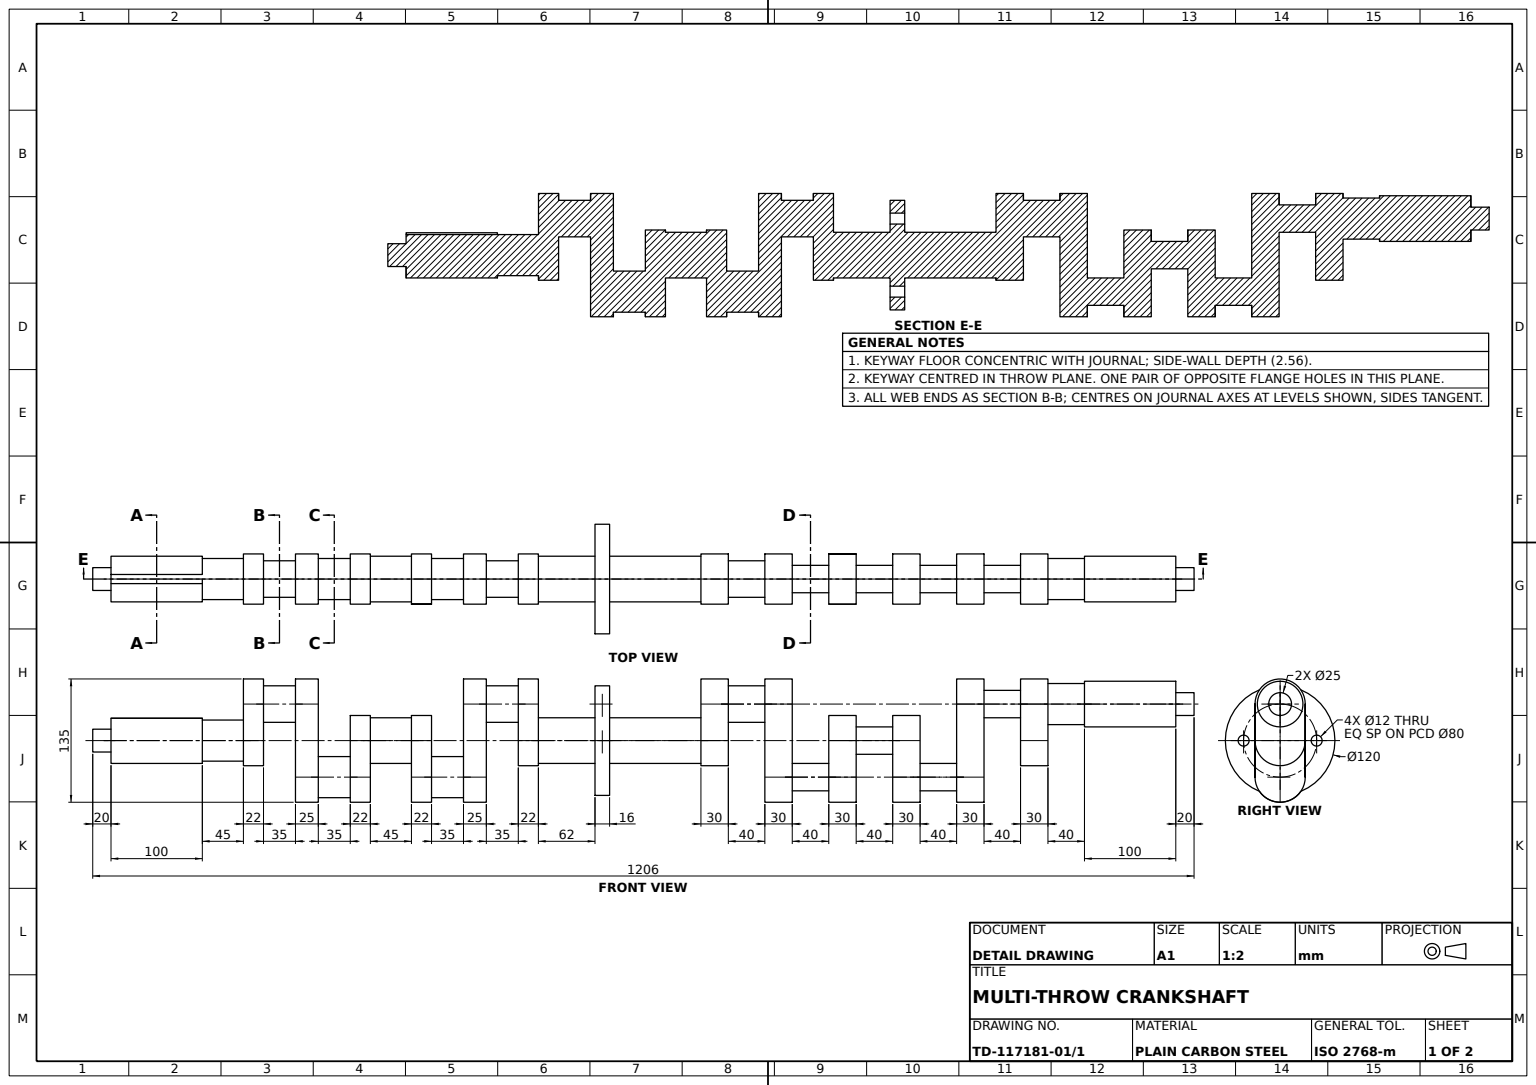
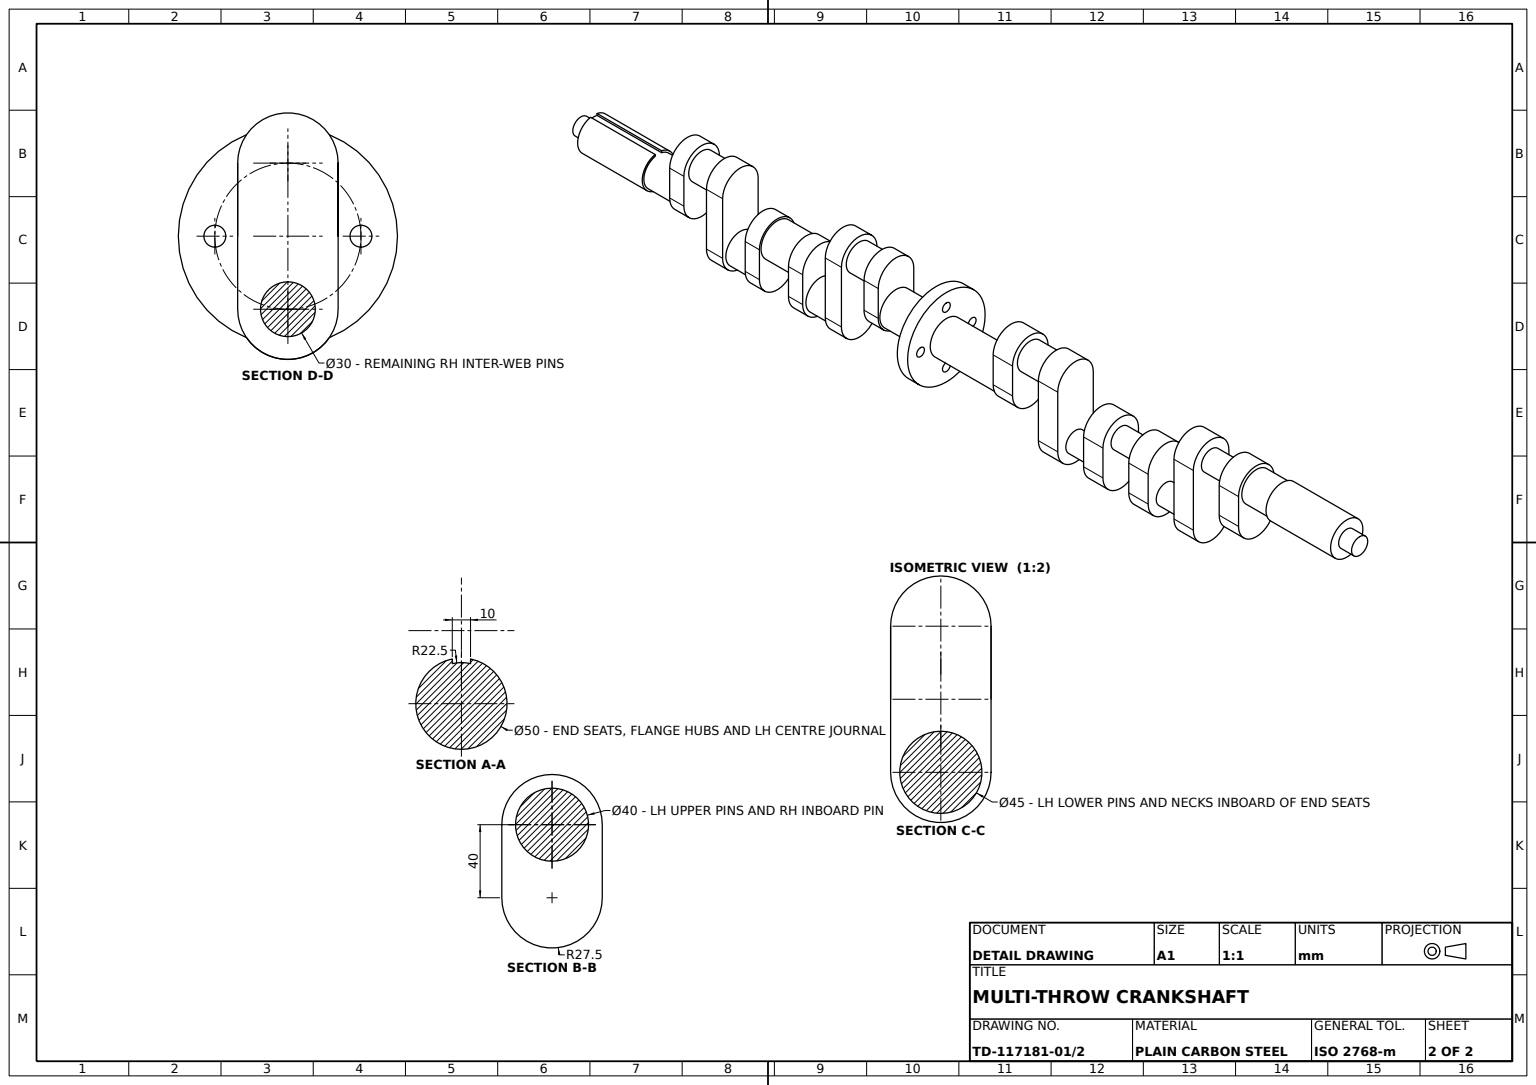
solid
v1 (0,-27.5,-240)
v2 (0,27.5,-240)
e1 v1 v2 CIRCLE(AX(P(0,0,-240),D(0,0,-1),D(-1,0,0)),27.5)
v3 (0,27.5,-270)
e2 v3 v2 LINE
v4 (0,-27.5,-270)
e3 v4 v3 CIRCLE(AX(P(0,0,-270),D(0,0,-1),D(-1,0,0)),27.5)
e4 v4 v1 LINE
face CYL(AX(P(0,0,-270),D(0,0,1),D(1,0,0)),27.5) [e1 -e2 -e3 e4]
v5 (62.5,0,195)
v6 (62.5,0,160)
e5 v5 v6 LINE
v7 (17.5,0,160)
e6 v6 v7 CIRCLE(AX(P(40,0,160),D(0,0,1),D(1,0,0)),22.5)
v8 (17.5,0,195)
e7 v8 v7 LINE
e8 v5 v8 CIRCLE(AX(P(40,0,195),D(0,0,1),D(1,0,0)),22.5)
face CYL(AX(P(40,0,195),D(0,0,-1),D(-1,0,0)),22.5) [e5 e6 -e7 -e8]
v9 (-25,0,-410)
v10 (-55,0,-410)
e9 v9 v10 CIRCLE(AX(P(-40,0,-410),D(0,0,-1),D(-1,0,0)),15)
v11 (-55,0,-450)
e10 v11 v10 LINE
v12 (-25,0,-450)
e11 v12 v11 CIRCLE(AX(P(-40,0,-450),D(0,0,-1),D(-1,0,0)),15)
e12 v12 v9 LINE
face CYL(AX(P(-40,0,-450),D(0,0,1),D(1,0,0)),15) [e9 -e10 -e11 e12]
v13 (-40,27.5,78)
v14 (-67.5,0,78)
e13 v13 v14 CIRCLE(AX(P(-40,0,78),D(0,0,1),D(1,0,0)),27.5)
v15 (-67.5,0,100)
e14 v15 v14 LINE
v16 (-40,27.5,100)
e15 v16 v15 CIRCLE(AX(P(-40,0,100),D(0,0,1),D(1,0,0)),27.5)
e16 v16 v13 LINE
face CYL(AX(P(-40,0,100),D(0,0,-1),D(-1,0,0)),27.5) [e13 -e14 -e15 e16]
v17 (25,0,-240)
v18 (55,0,-240)
e17 v17 v18 CIRCLE(AX(P(40,0,-240),D(0,0,-1),D(-1,0,0)),15)
v19 (25,0,-200)
e18 v17 v19 LINE
v20 (55,0,-200)
e19 v19 v20 CIRCLE(AX(P(40,0,-200),D(0,0,-1),D(-1,0,0)),15)
e20 v18 v20 LINE
face CYL(AX(P(40,0,-240),D(0,0,1),D(1,0,0)),15) [-e17 e18 e19 -e20]
v21 (40,-27.5,160)
v22 (40,-27.5,135)
e21 v21 v22 LINE
v23 (-40,-27.5,160)
e22 v23 v21 LINE
v24 (-40,-27.5,135)
e23 v23 v24 LINE
e24 v24 v22 LINE
face PLANE(AX(P(-40,-27.5,160),D(0,1,0),D(0,0,1))) rev [-e21 -e22 e23 e24]
v25 (40,27.5,284)
v26 (40,27.5,262)
e25 v25 v26 LINE
v27 (40,-27.5,284)
e26 v27 v25 CIRCLE(AX(P(40,0,284),D(0,0,1),D(1,0,0)),27.5)
v28 (40,-27.5,262)
e27 v27 v28 LINE
e28 v28 v26 CIRCLE(AX(P(40,0,262),D(0,0,1),D(1,0,0)),27.5)
face CYL(AX(P(40,0,284),D(0,0,-1),D(-1,0,0)),27.5) [-e25 -e26 e27 e28]
v29 (0,27.5,401)
v30 (-40,27.5,401)
e29 v29 v30 LINE
v31 (0,27.5,379)
e30 v29 v31 LINE
v32 (-40,27.5,379)
e31 v31 v32 LINE
e32 v30 v32 LINE
face PLANE(AX(P(-40,27.5,401),D(0,-1,0),D(0,0,-1))) rev [-e29 e30 e31 -e32]
v33 (-34,0,16)
v34 (-46,0,16)
e33 v33 v34 CIRCLE(AX(P(-40,0,16),D(0,0,1),D(1,0,0)),6)
v35 (-46,0,0)
e34 v35 v34 LINE
v36 (-34,0,0)
e35 v36 v35 CIRCLE(AX(P(-40,0,0),D(0,0,1),D(1,0,0)),6)
e36 v36 v33 LINE
face CYL(AX(P(-40,0,0),D(0,0,1),D(1,0,0)),6) rev [e33 -e34 -e35 e36]
v37 (0,-27.5,-480)
v38 (-40,-27.5,-480)
e37 v37 v38 LINE
v39 (-40,27.5,-480)
e38 v38 v39 CIRCLE(AX(P(-40,0,-480),D(0,0,-1),D(-1,0,0)),27.5)
v40 (0,27.5,-480)
e39 v39 v40 LINE
v41 (27.5,0,-480)
e40 v40 v41 CIRCLE(AX(P(0,0,-480),D(0,0,-1),D(-1,0,0)),27.5)
e41 v41 v37 CIRCLE(AX(P(0,0,-480),D(0,0,-1),D(-1,0,0)),27.5)
v42 (-17.5,0,-480)
v43 (-62.5,0,-480)
e42 v42 v43 CIRCLE(AX(P(-40,0,-480),D(0,0,-1),D(-1,0,0)),22.5)
e43 v43 v42 CIRCLE(AX(P(-40,0,-480),D(0,0,-1),D(-1,0,0)),22.5)
face PLANE(AX(P(-40,0,-480),D(0,0,-1),D(-1,0,0))) [e37 e38 e39 e40 e41] [-e42 -e43]
e44 v11 v12 CIRCLE(AX(P(-40,0,-450),D(0,0,-1),D(-1,0,0)),15)
v44 (-40,-27.5,-450)
v45 (-40,27.5,-450)
e45 v44 v45 CIRCLE(AX(P(-40,0,-450),D(0,0,-1),D(-1,0,0)),27.5)
v46 (0,-27.5,-450)
e46 v46 v44 LINE
v47 (27.5,0,-450)
e47 v47 v46 CIRCLE(AX(P(0,0,-450),D(0,0,-1),D(-1,0,0)),27.5)
v48 (0,27.5,-450)
e48 v48 v47 CIRCLE(AX(P(0,0,-450),D(0,0,-1),D(-1,0,0)),27.5)
e49 v45 v48 LINE
face PLANE(AX(P(-40,0,-450),D(0,0,-1),D(-1,0,0))) rev [e44 e11] [-e45 -e46 -e47 -e48 -e49]
v49 (-15,0,-520)
v50 (-65,0,-520)
e50 v49 v50 CIRCLE(AX(P(-40,0,-520),D(0,0,-1),D(-1,0,0)),25)
v51 (-65,0,-620)
e51 v51 v50 LINE
v52 (-15,0,-620)
e52 v52 v51 CIRCLE(AX(P(-40,0,-620),D(0,0,-1),D(-1,0,0)),25)
e53 v52 v49 LINE
face CYL(AX(P(-40,0,-620),D(0,0,1),D(1,0,0)),25) [e50 -e51 -e52 e53]
v53 (-40,27.5,135)
v54 (-67.5,0,135)
e54 v53 v54 CIRCLE(AX(P(-40,0,135),D(0,0,1),D(1,0,0)),27.5)
v55 (-67.5,0,160)
e55 v55 v54 LINE
v56 (-40,27.5,160)
e56 v56 v55 CIRCLE(AX(P(-40,0,160),D(0,0,1),D(1,0,0)),27.5)
e57 v56 v53 LINE
face CYL(AX(P(-40,0,160),D(0,0,-1),D(-1,0,0)),27.5) [e54 -e55 -e56 e57]
v57 (40,27.5,-240)
v58 (67.5,0,-240)
e58 v57 v58 CIRCLE(AX(P(40,0,-240),D(0,0,-1),D(-1,0,0)),27.5)
v59 (67.5,0,-270)
e59 v59 v58 LINE
v60 (40,27.5,-270)
e60 v60 v59 CIRCLE(AX(P(40,0,-270),D(0,0,-1),D(-1,0,0)),27.5)
e61 v60 v57 LINE
face CYL(AX(P(40,0,-270),D(0,0,1),D(1,0,0)),27.5) [e58 -e59 -e60 e61]
e62 v10 v9 CIRCLE(AX(P(-40,0,-410),D(0,0,-1),D(-1,0,0)),15)
face CYL(AX(P(-40,0,-450),D(0,0,1),D(1,0,0)),15) [-e44 e10 e62 -e12]
v61 (40,-27.5,-240)
e63 v58 v61 CIRCLE(AX(P(40,0,-240),D(0,0,-1),D(-1,0,0)),27.5)
v62 (40,-27.5,-270)
e64 v62 v61 LINE
e65 v59 v62 CIRCLE(AX(P(40,0,-270),D(0,0,-1),D(-1,0,0)),27.5)
face CYL(AX(P(40,0,-270),D(0,0,1),D(1,0,0)),27.5) [e63 -e64 -e65 e59]
v63 (40,27.5,160)
e66 v21 v63 CIRCLE(AX(P(40,0,160),D(0,0,1),D(1,0,0)),27.5)
e67 v63 v56 LINE
e68 v55 v23 CIRCLE(AX(P(-40,0,160),D(0,0,1),D(1,0,0)),27.5)
e69 v7 v6 CIRCLE(AX(P(40,0,160),D(0,0,1),D(1,0,0)),22.5)
face PLANE(AX(P(-40,0,160),D(0,0,1),D(1,0,0))) [e66 e67 e56 e68 e22] [-e69 -e6]
v64 (-6,-40,0)
v65 (-6,-40,16)
e70 v64 v65 LINE
v66 (6,-40,0)
e71 v66 v64 CIRCLE(AX(P(0,-40,0),D(0,0,1),D(1,0,0)),6)
v67 (6,-40,16)
e72 v66 v67 LINE
e73 v67 v65 CIRCLE(AX(P(0,-40,16),D(0,0,1),D(1,0,0)),6)
face CYL(AX(P(0,-40,0),D(0,0,1),D(1,0,0)),6) rev [-e70 -e71 e72 e73]
v68 (55,0,-340)
v69 (25,0,-340)
e74 v68 v69 CIRCLE(AX(P(40,0,-340),D(0,0,-1),D(-1,0,0)),15)
v70 (25,0,-380)
e75 v70 v69 LINE
v71 (55,0,-380)
e76 v71 v70 CIRCLE(AX(P(40,0,-380),D(0,0,-1),D(-1,0,0)),15)
e77 v71 v68 LINE
face CYL(AX(P(40,0,-380),D(0,0,1),D(1,0,0)),15) [e74 -e75 -e76 e77]
v72 (-20,0,-130)
v73 (-60,0,-130)
e78 v72 v73 CIRCLE(AX(P(-40,0,-130),D(0,0,-1),D(-1,0,0)),20)
e79 v73 v72 CIRCLE(AX(P(-40,0,-130),D(0,0,-1),D(-1,0,0)),20)
v74 (0,-27.5,-130)
v75 (-40,-27.5,-130)
e80 v74 v75 LINE
v76 (-40,27.5,-130)
e81 v75 v76 CIRCLE(AX(P(-40,0,-130),D(0,0,-1),D(-1,0,0)),27.5)
v77 (0,27.5,-130)
e82 v76 v77 LINE
v78 (27.5,0,-130)
e83 v77 v78 CIRCLE(AX(P(0,0,-130),D(0,0,-1),D(-1,0,0)),27.5)
e84 v78 v74 CIRCLE(AX(P(0,0,-130),D(0,0,-1),D(-1,0,0)),27.5)
face PLANE(AX(P(0,0,-130),D(0,0,-1),D(-1,0,0))) [-e78 -e79] [e80 e81 e82 e83 e84]
v79 (15,0,-310)
v80 (-15,0,-310)
e85 v79 v80 CIRCLE(AX(P(0,0,-310),D(0,0,-1),D(-1,0,0)),15)
e86 v80 v79 CIRCLE(AX(P(0,0,-310),D(0,0,-1),D(-1,0,0)),15)
v81 (40,-27.5,-310)
v82 (0,-27.5,-310)
e87 v81 v82 LINE
v83 (67.5,0,-310)
e88 v83 v81 CIRCLE(AX(P(40,0,-310),D(0,0,-1),D(-1,0,0)),27.5)
v84 (40,27.5,-310)
e89 v84 v83 CIRCLE(AX(P(40,0,-310),D(0,0,-1),D(-1,0,0)),27.5)
v85 (0,27.5,-310)
e90 v85 v84 LINE
e91 v82 v85 CIRCLE(AX(P(0,0,-310),D(0,0,-1),D(-1,0,0)),27.5)
face PLANE(AX(P(0,0,-310),D(0,0,-1),D(-1,0,0))) rev [e85 e86] [-e87 -e88 -e89 -e90 -e91]
v86 (-12.5,0,546)
v87 (12.5,0,546)
e92 v86 v87 CIRCLE(AX(P(0,0,546),D(0,0,1),D(1,0,0)),12.5)
v88 (12.5,0,566)
e93 v88 v87 LINE
v89 (-12.5,0,566)
e94 v89 v88 CIRCLE(AX(P(0,0,566),D(0,0,1),D(1,0,0)),12.5)
e95 v89 v86 LINE
face CYL(AX(P(0,0,566),D(0,0,-1),D(-1,0,0)),12.5) [e92 -e93 -e94 e95]
v90 (-20,0,-170)
v91 (-60,0,-170)
e96 v90 v91 CIRCLE(AX(P(-40,0,-170),D(0,0,-1),D(-1,0,0)),20)
e97 v90 v72 LINE
e98 v91 v73 LINE
face CYL(AX(P(-40,0,-170),D(0,0,1),D(1,0,0)),20) [-e96 e97 e78 -e98]
v92 (15,0,-270)
e99 v79 v92 LINE
v93 (-15,0,-270)
e100 v92 v93 CIRCLE(AX(P(0,0,-270),D(0,0,-1),D(-1,0,0)),15)
e101 v80 v93 LINE
face CYL(AX(P(0,0,-310),D(0,0,1),D(1,0,0)),15) [-e85 e99 e100 -e101]
v94 (0,-27.5,100)
v95 (0,27.5,100)
e102 v94 v95 CIRCLE(AX(P(0,0,100),D(0,0,1),D(1,0,0)),27.5)
v96 (0,-27.5,78)
e103 v94 v96 LINE
v97 (0,27.5,78)
e104 v96 v97 CIRCLE(AX(P(0,0,78),D(0,0,1),D(1,0,0)),27.5)
e105 v95 v97 LINE
face CYL(AX(P(0,0,100),D(0,0,-1),D(-1,0,0)),27.5) [-e102 e103 e104 -e105]
v98 (-52.5,0,-640)
v99 (-27.5,0,-640)
e106 v98 v99 CIRCLE(AX(P(-40,0,-640),D(0,0,-1),D(-1,0,0)),12.5)
v100 (-52.5,0,-620)
e107 v98 v100 LINE
v101 (-27.5,0,-620)
e108 v100 v101 CIRCLE(AX(P(-40,0,-620),D(0,0,-1),D(-1,0,0)),12.5)
e109 v99 v101 LINE
face CYL(AX(P(-40,0,-640),D(0,0,1),D(1,0,0)),12.5) [-e106 e107 e108 -e109]
v102 (-22.5,0,401)
v103 (22.5,0,401)
e110 v102 v103 CIRCLE(AX(P(0,0,401),D(0,0,1),D(1,0,0)),22.5)
e111 v103 v102 CIRCLE(AX(P(0,0,401),D(0,0,1),D(1,0,0)),22.5)
v104 (-40,-27.5,401)
v105 (0,-27.5,401)
e112 v104 v105 LINE
e113 v105 v29 CIRCLE(AX(P(0,0,401),D(0,0,1),D(1,0,0)),27.5)
v106 (-67.5,0,401)
e114 v30 v106 CIRCLE(AX(P(-40,0,401),D(0,0,1),D(1,0,0)),27.5)
e115 v106 v104 CIRCLE(AX(P(-40,0,401),D(0,0,1),D(1,0,0)),27.5)
face PLANE(AX(P(-40,0,401),D(0,0,1),D(1,0,0))) [-e110 -e111] [e112 e113 e29 e114 e115]
v107 (60,0,0)
v108 (-60,0,0)
e116 v107 v108 CIRCLE(AX(P(0,0,0),D(0,0,1),D(1,0,0)),60)
v109 (-60,0,16)
e117 v109 v108 LINE
v110 (60,0,16)
e118 v110 v109 CIRCLE(AX(P(0,0,16),D(0,0,1),D(1,0,0)),60)
e119 v110 v107 LINE
face CYL(AX(P(0,0,16),D(0,0,-1),D(-1,0,0)),60) [e116 -e117 -e118 e119]
v111 (0,-27.5,379)
e120 v105 v111 LINE
e121 v111 v31 CIRCLE(AX(P(0,0,379),D(0,0,1),D(1,0,0)),27.5)
face CYL(AX(P(0,0,401),D(0,0,-1),D(-1,0,0)),27.5) [-e113 e120 e121 -e30]
e122 v95 v16 LINE
e123 v97 v13 LINE
face PLANE(AX(P(0,27.5,100),D(0,-1,0),D(1,0,0))) rev [-e122 e105 e123 -e16]
v112 (40,27.5,195)
v113 (0,27.5,195)
e124 v112 v113 LINE
v114 (0,27.5,217)
e125 v114 v113 LINE
v115 (40,27.5,217)
e126 v115 v114 LINE
e127 v115 v112 LINE
face PLANE(AX(P(40,27.5,217),D(0,-1,0),D(1,0,0))) rev [e124 -e125 -e126 e127]
v116 (27.5,0,-100)
e128 v78 v116 LINE
v117 (0,-27.5,-100)
e129 v116 v117 CIRCLE(AX(P(0,0,-100),D(0,0,-1),D(-1,0,0)),27.5)
e130 v74 v117 LINE
face CYL(AX(P(0,0,-130),D(0,0,1),D(1,0,0)),27.5) [-e84 e128 e129 -e130]
e131 v37 v46 LINE
e132 v41 v47 LINE
face CYL(AX(P(0,0,-480),D(0,0,1),D(1,0,0)),27.5) [e47 -e131 -e41 e132]
v118 (40,-27.5,-340)
v119 (0,-27.5,-340)
e133 v118 v119 LINE
v120 (0,27.5,-340)
e134 v119 v120 CIRCLE(AX(P(0,0,-340),D(0,0,-1),D(-1,0,0)),27.5)
v121 (40,27.5,-340)
e135 v120 v121 LINE
v122 (67.5,0,-340)
e136 v121 v122 CIRCLE(AX(P(40,0,-340),D(0,0,-1),D(-1,0,0)),27.5)
e137 v122 v118 CIRCLE(AX(P(40,0,-340),D(0,0,-1),D(-1,0,0)),27.5)
e138 v69 v68 CIRCLE(AX(P(40,0,-340),D(0,0,-1),D(-1,0,0)),15)
face PLANE(AX(P(0,0,-340),D(0,0,-1),D(-1,0,0))) [e133 e134 e135 e136 e137] [-e74 -e138]
v123 (0,27.5,-100)
e139 v77 v123 LINE
v124 (-40,27.5,-100)
e140 v76 v124 LINE
e141 v124 v123 LINE
face PLANE(AX(P(0,27.5,-130),D(0,-1,0),D(0,0,-1))) rev [-e139 -e82 e140 e141]
v125 (40,-27.5,319)
v126 (40,27.5,319)
e142 v125 v126 CIRCLE(AX(P(40,0,319),D(0,0,1),D(1,0,0)),27.5)
v127 (40,27.5,344)
e143 v127 v126 LINE
v128 (40,-27.5,344)
e144 v128 v127 CIRCLE(AX(P(40,0,344),D(0,0,1),D(1,0,0)),27.5)
e145 v128 v125 LINE
face CYL(AX(P(40,0,344),D(0,0,-1),D(-1,0,0)),27.5) [e142 -e143 -e144 e145]
e146 v54 v24 CIRCLE(AX(P(-40,0,135),D(0,0,1),D(1,0,0)),27.5)
face CYL(AX(P(-40,0,160),D(0,0,-1),D(-1,0,0)),27.5) [e146 -e23 -e68 e55]
v129 (-40,27.5,-410)
v130 (40,27.5,-410)
e147 v129 v130 LINE
v131 (67.5,0,-410)
e148 v130 v131 CIRCLE(AX(P(40,0,-410),D(0,0,-1),D(-1,0,0)),27.5)
v132 (40,-27.5,-410)
e149 v131 v132 CIRCLE(AX(P(40,0,-410),D(0,0,-1),D(-1,0,0)),27.5)
v133 (-40,-27.5,-410)
e150 v132 v133 LINE
e151 v133 v129 CIRCLE(AX(P(-40,0,-410),D(0,0,-1),D(-1,0,0)),27.5)
face PLANE(AX(P(40,0,-410),D(0,0,-1),D(-1,0,0))) [-e9 -e62] [e147 e148 e149 e150 e151]
v134 (40,-27.5,-380)
e152 v132 v134 LINE
v135 (67.5,0,-380)
e153 v131 v135 LINE
e154 v135 v134 CIRCLE(AX(P(40,0,-380),D(0,0,-1),D(-1,0,0)),27.5)
face CYL(AX(P(40,0,-410),D(0,0,1),D(1,0,0)),27.5) [-e152 -e149 e153 e154]
v136 (-27.5,0,284)
v137 (-27.5,0,262)
e155 v136 v137 LINE
v138 (0,27.5,284)
e156 v138 v136 CIRCLE(AX(P(0,0,284),D(0,0,1),D(1,0,0)),27.5)
v139 (0,27.5,262)
e157 v138 v139 LINE
e158 v139 v137 CIRCLE(AX(P(0,0,262),D(0,0,1),D(1,0,0)),27.5)
face CYL(AX(P(0,0,284),D(0,0,-1),D(-1,0,0)),27.5) [-e155 -e156 e157 e158]
v140 (62.5,0,319)
v141 (62.5,0,284)
e159 v140 v141 LINE
v142 (17.5,0,319)
e160 v142 v140 CIRCLE(AX(P(40,0,319),D(0,0,1),D(1,0,0)),22.5)
v143 (17.5,0,284)
e161 v142 v143 LINE
e162 v143 v141 CIRCLE(AX(P(40,0,284),D(0,0,1),D(1,0,0)),22.5)
face CYL(AX(P(40,0,319),D(0,0,-1),D(-1,0,0)),22.5) [-e159 -e160 e161 e162]
e163 v101 v100 CIRCLE(AX(P(-40,0,-620),D(0,0,-1),D(-1,0,0)),12.5)
e164 v51 v52 CIRCLE(AX(P(-40,0,-620),D(0,0,-1),D(-1,0,0)),25)
face PLANE(AX(P(-40,0,-620),D(0,0,-1),D(-1,0,0))) [-e163 -e108] [e52 e164]
e165 v121 v84 LINE
e166 v122 v83 LINE
face CYL(AX(P(40,0,-340),D(0,0,1),D(1,0,0)),27.5) [e165 e89 -e166 -e136]
v144 (0,-27.5,217)
v145 (0,-27.5,195)
e167 v144 v145 LINE
v146 (40,-27.5,195)
e168 v145 v146 LINE
v147 (40,-27.5,217)
e169 v147 v146 LINE
e170 v144 v147 LINE
face PLANE(AX(P(40,-27.5,217),D(0,1,0),D(0,0,1))) rev [e167 e168 -e169 -e170]
v148 (-24.494897,-5,546)
v149 (-24.494897,-5,446)
e171 v148 v149 LINE
v150 (-21.937411,-5,546)
e172 v150 v148 LINE
v151 (-21.937411,-5,446)
e173 v150 v151 LINE
e174 v151 v149 LINE
face PLANE(AX(P(-21.937411,-5,546),D(0,-1,0),D(1,0,0))) rev [-e171 -e172 e173 e174]
v152 (-24.494897,5,546)
e175 v148 v152 CIRCLE(AX(P(0,0,546),D(0,0,1),D(1,0,0)),25)
v153 (-21.937411,5,546)
e176 v152 v153 LINE
v154 (-22.5,0,546)
e177 v153 v154 CIRCLE(AX(P(0,0,546),D(0,0,1),D(1,0,0)),22.5)
e178 v154 v150 CIRCLE(AX(P(0,0,546),D(0,0,1),D(1,0,0)),22.5)
e179 v87 v86 CIRCLE(AX(P(0,0,546),D(0,0,1),D(1,0,0)),12.5)
face PLANE(AX(P(0,0,546),D(0,0,1),D(1,0,0))) [e175 e176 e177 e178 e172] [-e92 -e179]
v155 (-40,-27.5,100)
e180 v15 v155 CIRCLE(AX(P(-40,0,100),D(0,0,1),D(1,0,0)),27.5)
e181 v155 v94 LINE
v156 (-60,0,100)
v157 (-20,0,100)
e182 v156 v157 CIRCLE(AX(P(-40,0,100),D(0,0,1),D(1,0,0)),20)
e183 v157 v156 CIRCLE(AX(P(-40,0,100),D(0,0,1),D(1,0,0)),20)
face PLANE(AX(P(0,0,100),D(0,0,1),D(1,0,0))) [e180 e181 e102 e122 e15] [-e182 -e183]
v158 (-40,27.5,344)
e184 v127 v158 LINE
v159 (-40,27.5,319)
e185 v126 v159 LINE
e186 v158 v159 LINE
face PLANE(AX(P(40,27.5,344),D(0,-1,0),D(1,0,0))) rev [-e184 e143 e185 -e186]
e187 v118 v81 LINE
e188 v119 v82 LINE
face PLANE(AX(P(0,-27.5,-340),D(0,1,0),D(0,0,1))) rev [-e133 e187 e87 -e188]
v160 (-60,0,379)
v161 (-60,0,344)
e189 v160 v161 LINE
v162 (-20,0,344)
e190 v161 v162 CIRCLE(AX(P(-40,0,344),D(0,0,1),D(1,0,0)),20)
v163 (-20,0,379)
e191 v163 v162 LINE
e192 v160 v163 CIRCLE(AX(P(-40,0,379),D(0,0,1),D(1,0,0)),20)
face CYL(AX(P(-40,0,379),D(0,0,-1),D(-1,0,0)),20) [e189 e190 -e191 -e192]
e193 v62 v4 LINE
e194 v3 v60 LINE
e195 v93 v92 CIRCLE(AX(P(0,0,-270),D(0,0,-1),D(-1,0,0)),15)
face PLANE(AX(P(40,0,-270),D(0,0,-1),D(-1,0,0))) [e193 e3 e194 e60 e65] [-e195 -e100]
e196 v140 v142 CIRCLE(AX(P(40,0,319),D(0,0,1),D(1,0,0)),22.5)
v164 (-40,-27.5,319)
e197 v164 v125 LINE
v165 (-67.5,0,319)
e198 v165 v164 CIRCLE(AX(P(-40,0,319),D(0,0,1),D(1,0,0)),27.5)
e199 v159 v165 CIRCLE(AX(P(-40,0,319),D(0,0,1),D(1,0,0)),27.5)
face PLANE(AX(P(40,0,319),D(0,0,1),D(1,0,0))) rev [e160 e196] [-e185 -e142 -e197 -e198 -e199]
v166 (34,0,0)
v167 (46,0,0)
e200 v166 v167 CIRCLE(AX(P(40,0,0),D(0,0,1),D(1,0,0)),6)
v168 (34,0,16)
e201 v166 v168 LINE
v169 (46,0,16)
e202 v168 v169 CIRCLE(AX(P(40,0,16),D(0,0,1),D(1,0,0)),6)
e203 v167 v169 LINE
face CYL(AX(P(40,0,0),D(0,0,1),D(1,0,0)),6) rev [-e200 e201 e202 -e203]
e204 v50 v49 CIRCLE(AX(P(-40,0,-520),D(0,0,-1),D(-1,0,0)),25)
v170 (-62.5,0,-520)
v171 (-17.5,0,-520)
e205 v170 v171 CIRCLE(AX(P(-40,0,-520),D(0,0,-1),D(-1,0,0)),22.5)
e206 v171 v170 CIRCLE(AX(P(-40,0,-520),D(0,0,-1),D(-1,0,0)),22.5)
face PLANE(AX(P(-40,0,-520),D(0,0,-1),D(-1,0,0))) rev [-e50 -e204] [e205 e206]
v172 (40,27.5,135)
e207 v172 v53 LINE
e208 v22 v172 CIRCLE(AX(P(40,0,135),D(0,0,1),D(1,0,0)),27.5)
v173 (-20,0,135)
v174 (-60,0,135)
e209 v173 v174 CIRCLE(AX(P(-40,0,135),D(0,0,1),D(1,0,0)),20)
e210 v174 v173 CIRCLE(AX(P(-40,0,135),D(0,0,1),D(1,0,0)),20)
face PLANE(AX(P(-40,0,135),D(0,0,1),D(1,0,0))) rev [-e146 -e54 -e207 -e208 -e24] [e209 e210]
face CYL(AX(P(-40,0,-620),D(0,0,1),D(1,0,0)),25) [e204 -e53 -e164 e51]
v175 (-40,-27.5,-170)
v176 (-40,27.5,-170)
e211 v175 v176 CIRCLE(AX(P(-40,0,-170),D(0,0,-1),D(-1,0,0)),27.5)
v177 (-40,27.5,-200)
e212 v177 v176 LINE
v178 (-40,-27.5,-200)
e213 v178 v177 CIRCLE(AX(P(-40,0,-200),D(0,0,-1),D(-1,0,0)),27.5)
e214 v178 v175 LINE
face CYL(AX(P(-40,0,-200),D(0,0,1),D(1,0,0)),27.5) [e211 -e212 -e213 e214]
v179 (-25,0,78)
v180 (-25,0,16)
e215 v179 v180 LINE
v181 (25,0,78)
e216 v181 v179 CIRCLE(AX(P(0,0,78),D(0,0,1),D(1,0,0)),25)
v182 (25,0,16)
e217 v181 v182 LINE
e218 v182 v180 CIRCLE(AX(P(0,0,16),D(0,0,1),D(1,0,0)),25)
face CYL(AX(P(0,0,78),D(0,0,-1),D(-1,0,0)),25) [-e215 -e216 e217 e218]
e219 v99 v98 CIRCLE(AX(P(-40,0,-640),D(0,0,-1),D(-1,0,0)),12.5)
face PLANE(AX(P(-40,0,-640),D(0,0,-1),D(-1,0,0))) [e106 e219]
e220 v40 v48 LINE
e221 v39 v45 LINE
face PLANE(AX(P(-40,27.5,-480),D(0,-1,0),D(1,0,0))) rev [-e220 -e39 e221 e49]
e222 v174 v156 LINE
e223 v173 v157 LINE
face CYL(AX(P(-40,0,135),D(0,0,-1),D(-1,0,0)),20) [e222 e182 -e223 -e210]
e224 v34 v33 CIRCLE(AX(P(-40,0,16),D(0,0,1),D(1,0,0)),6)
e225 v180 v182 CIRCLE(AX(P(0,0,16),D(0,0,1),D(1,0,0)),25)
e226 v109 v110 CIRCLE(AX(P(0,0,16),D(0,0,1),D(1,0,0)),60)
v183 (-6,40,16)
v184 (6,40,16)
e227 v183 v184 CIRCLE(AX(P(0,40,16),D(0,0,1),D(1,0,0)),6)
e228 v184 v183 CIRCLE(AX(P(0,40,16),D(0,0,1),D(1,0,0)),6)
e229 v65 v67 CIRCLE(AX(P(0,-40,16),D(0,0,1),D(1,0,0)),6)
e230 v169 v168 CIRCLE(AX(P(40,0,16),D(0,0,1),D(1,0,0)),6)
face PLANE(AX(P(0,0,16),D(0,0,1),D(1,0,0))) [-e33 -e224] [-e218 -e225] [e118 e226] [-e227 -e228] [-e229 -e73] [-e202 -e230]
e231 v154 v102 LINE
v185 (22.5,0,446)
e232 v185 v103 LINE
e233 v151 v185 CIRCLE(AX(P(0,0,446),D(0,0,1),D(1,0,0)),22.5)
face CYL(AX(P(0,0,446),D(0,0,-1),D(-1,0,0)),22.5) [-e173 -e178 e231 e110 -e232 -e233]
e234 v8 v5 CIRCLE(AX(P(40,0,195),D(0,0,1),D(1,0,0)),22.5)
face CYL(AX(P(40,0,195),D(0,0,-1),D(-1,0,0)),22.5) [-e5 -e234 e7 e69]
v186 (40,27.5,-200)
v187 (67.5,0,-200)
e235 v186 v187 CIRCLE(AX(P(40,0,-200),D(0,0,-1),D(-1,0,0)),27.5)
v188 (40,27.5,-170)
e236 v186 v188 LINE
v189 (67.5,0,-170)
e237 v188 v189 CIRCLE(AX(P(40,0,-170),D(0,0,-1),D(-1,0,0)),27.5)
e238 v187 v189 LINE
face CYL(AX(P(40,0,-200),D(0,0,1),D(1,0,0)),27.5) [-e235 e236 e237 -e238]
v190 (-40,-27.5,-100)
e239 v117 v190 LINE
e240 v75 v190 LINE
face PLANE(AX(P(0,-27.5,-130),D(0,1,0),D(0,0,1))) rev [e239 -e240 -e80 e130]
e241 v35 v36 CIRCLE(AX(P(-40,0,0),D(0,0,1),D(1,0,0)),6)
face CYL(AX(P(-40,0,0),D(0,0,1),D(1,0,0)),6) rev [e34 e224 -e36 -e241]
v191 (0,-27.5,262)
e242 v191 v28 LINE
v192 (0,-27.5,284)
e243 v192 v27 LINE
e244 v192 v191 LINE
face PLANE(AX(P(0,-27.5,284),D(0,1,0),D(0,0,1))) rev [e242 -e27 -e243 e244]
v193 (40,27.5,-380)
e245 v130 v193 LINE
v194 (-40,27.5,-380)
e246 v129 v194 LINE
e247 v194 v193 LINE
face PLANE(AX(P(40,27.5,-410),D(0,-1,0),D(0,0,-1))) rev [-e245 -e147 e246 e247]
v195 (25,0,-100)
v196 (25,0,0)
e248 v195 v196 LINE
v197 (-25,0,-100)
e249 v197 v195 CIRCLE(AX(P(0,0,-100),D(0,0,-1),D(-1,0,0)),25)
v198 (-25,0,0)
e250 v197 v198 LINE
e251 v198 v196 CIRCLE(AX(P(0,0,0),D(0,0,-1),D(1,0,0)),25)
face CYL(AX(P(0,0,-100),D(0,0,1),D(1,0,0)),25) [-e248 -e249 e250 e251]
v199 (-40,-27.5,78)
e252 v155 v199 LINE
e253 v14 v199 CIRCLE(AX(P(-40,0,78),D(0,0,1),D(1,0,0)),27.5)
face CYL(AX(P(-40,0,100),D(0,0,-1),D(-1,0,0)),27.5) [-e252 -e180 e14 e253]
v200 (-40,-27.5,-380)
e254 v134 v200 LINE
e255 v133 v200 LINE
face PLANE(AX(P(40,-27.5,-410),D(0,1,0),D(0,0,1))) rev [e152 e254 -e255 -e150]
face CYL(AX(P(-40,0,135),D(0,0,-1),D(-1,0,0)),20) [e183 -e222 -e209 e223]
e256 v70 v71 CIRCLE(AX(P(40,0,-380),D(0,0,-1),D(-1,0,0)),15)
face CYL(AX(P(40,0,-380),D(0,0,1),D(1,0,0)),15) [e75 e138 -e77 -e256]
face CYL(AX(P(-40,0,-640),D(0,0,1),D(1,0,0)),12.5) [e163 -e107 -e219 e109]
face CYL(AX(P(0,0,-310),D(0,0,1),D(1,0,0)),15) [-e86 e101 e195 -e99]
v201 (-24.494897,5,446)
e257 v152 v201 LINE
v202 (-21.937411,5,446)
e258 v201 v202 LINE
e259 v153 v202 LINE
face PLANE(AX(P(-24.494897,5,546),D(0,1,0),D(-1,0,0))) rev [e257 e258 -e259 -e176]
e260 v38 v44 LINE
face PLANE(AX(P(-40,-27.5,-480),D(0,1,0),D(0,0,1))) rev [e131 e46 -e260 -e37]
v203 (-40,-27.5,379)
e261 v104 v203 LINE
e262 v203 v111 LINE
face PLANE(AX(P(-40,-27.5,401),D(0,1,0),D(0,0,1))) rev [-e120 -e112 e261 e262]
e263 v20 v19 CIRCLE(AX(P(40,0,-200),D(0,0,-1),D(-1,0,0)),15)
v204 (40,-27.5,-200)
e264 v204 v178 LINE
e265 v177 v186 LINE
e266 v187 v204 CIRCLE(AX(P(40,0,-200),D(0,0,-1),D(-1,0,0)),27.5)
face PLANE(AX(P(-40,0,-200),D(0,0,-1),D(-1,0,0))) [-e19 -e263] [e264 e213 e265 e235 e266]
e267 v162 v161 CIRCLE(AX(P(-40,0,344),D(0,0,1),D(1,0,0)),20)
e268 v163 v160 CIRCLE(AX(P(-40,0,379),D(0,0,1),D(1,0,0)),20)
face CYL(AX(P(-40,0,379),D(0,0,-1),D(-1,0,0)),20) [e267 -e189 -e268 e191]
e269 v179 v181 CIRCLE(AX(P(0,0,78),D(0,0,1),D(1,0,0)),25)
face CYL(AX(P(0,0,78),D(0,0,-1),D(-1,0,0)),25) [e225 -e217 -e269 e215]
e270 v61 v1 LINE
face PLANE(AX(P(40,-27.5,-270),D(0,1,0),D(0,0,1))) rev [e64 e270 -e4 -e193]
v205 (-67.5,0,379)
e271 v106 v205 LINE
e272 v32 v205 CIRCLE(AX(P(-40,0,379),D(0,0,1),D(1,0,0)),27.5)
face CYL(AX(P(-40,0,401),D(0,0,-1),D(-1,0,0)),27.5) [-e271 -e114 e32 e272]
v206 (-27.5,0,217)
e273 v206 v144 CIRCLE(AX(P(0,0,217),D(0,0,1),D(1,0,0)),27.5)
v207 (-27.5,0,195)
e274 v206 v207 LINE
e275 v207 v145 CIRCLE(AX(P(0,0,195),D(0,0,1),D(1,0,0)),27.5)
face CYL(AX(P(0,0,217),D(0,0,-1),D(-1,0,0)),27.5) [-e273 e274 e275 -e167]
v208 (25,0,262)
v209 (-25,0,262)
e276 v208 v209 CIRCLE(AX(P(0,0,262),D(0,0,1),D(1,0,0)),25)
e277 v209 v208 CIRCLE(AX(P(0,0,262),D(0,0,1),D(1,0,0)),25)
e278 v137 v191 CIRCLE(AX(P(0,0,262),D(0,0,1),D(1,0,0)),27.5)
e279 v26 v139 LINE
face PLANE(AX(P(0,0,262),D(0,0,1),D(1,0,0))) rev [e276 e277] [-e278 -e158 -e279 -e28 -e242]
v210 (25,0,217)
v211 (-25,0,217)
e280 v210 v211 CIRCLE(AX(P(0,0,217),D(0,0,1),D(1,0,0)),25)
e281 v209 v211 LINE
e282 v208 v210 LINE
face CYL(AX(P(0,0,262),D(0,0,-1),D(-1,0,0)),25) [e280 -e281 -e276 e282]
e283 v185 v202 CIRCLE(AX(P(0,0,446),D(0,0,1),D(1,0,0)),22.5)
face CYL(AX(P(0,0,446),D(0,0,-1),D(-1,0,0)),22.5) [-e177 e259 -e283 e232 e111 -e231]
e284 v136 v192 CIRCLE(AX(P(0,0,284),D(0,0,1),D(1,0,0)),27.5)
e285 v25 v138 LINE
e286 v141 v143 CIRCLE(AX(P(40,0,284),D(0,0,1),D(1,0,0)),22.5)
face PLANE(AX(P(0,0,284),D(0,0,1),D(1,0,0))) [e156 e284 e243 e26 e285] [-e286 -e162]
e287 v199 v96 LINE
face PLANE(AX(P(0,-27.5,100),D(0,1,0),D(-1,0,0))) rev [e252 e287 -e103 -e181]
e288 v147 v115 CIRCLE(AX(P(40,0,217),D(0,0,1),D(1,0,0)),27.5)
e289 v146 v112 CIRCLE(AX(P(40,0,195),D(0,0,1),D(1,0,0)),27.5)
face CYL(AX(P(40,0,217),D(0,0,-1),D(-1,0,0)),27.5) [-e127 -e288 e169 e289]
e290 v64 v66 CIRCLE(AX(P(0,-40,0),D(0,0,1),D(1,0,0)),6)
face CYL(AX(P(0,-40,0),D(0,0,1),D(1,0,0)),6) rev [-e72 -e290 e70 e229]
e291 v176 v188 LINE
face PLANE(AX(P(-40,27.5,-200),D(0,-1,0),D(1,0,0))) rev [e291 -e236 -e265 e212]
v212 (6,40,0)
e292 v212 v184 LINE
v213 (-6,40,0)
e293 v213 v212 CIRCLE(AX(P(0,40,0),D(0,0,1),D(1,0,0)),6)
e294 v213 v183 LINE
face CYL(AX(P(0,40,0),D(0,0,1),D(1,0,0)),6) rev [e227 -e292 -e293 e294]
v214 (40,-27.5,-170)
e295 v204 v214 LINE
e296 v189 v214 CIRCLE(AX(P(40,0,-170),D(0,0,-1),D(-1,0,0)),27.5)
face CYL(AX(P(40,0,-200),D(0,0,1),D(1,0,0)),27.5) [-e295 -e266 e238 e296]
e297 v190 v124 CIRCLE(AX(P(-40,0,-100),D(0,0,-1),D(-1,0,0)),27.5)
face CYL(AX(P(-40,0,-130),D(0,0,1),D(1,0,0)),27.5) [-e81 e240 e297 -e140]
e298 v211 v210 CIRCLE(AX(P(0,0,217),D(0,0,1),D(1,0,0)),25)
face CYL(AX(P(0,0,262),D(0,0,-1),D(-1,0,0)),25) [-e277 e281 e298 -e282]
e299 v113 v207 CIRCLE(AX(P(0,0,195),D(0,0,1),D(1,0,0)),27.5)
face PLANE(AX(P(40,0,195),D(0,0,1),D(1,0,0))) rev [-e124 -e289 -e168 -e275 -e299] [e234 e8]
face CYL(AX(P(40,0,319),D(0,0,-1),D(-1,0,0)),22.5) [-e196 e159 e286 -e161]
e300 v88 v89 CIRCLE(AX(P(0,0,566),D(0,0,1),D(1,0,0)),12.5)
face PLANE(AX(P(0,0,566),D(0,0,1),D(1,0,0))) [e94 e300]
face CYL(AX(P(40,0,-340),D(0,0,1),D(1,0,0)),27.5) [e88 -e187 -e137 e166]
e301 v91 v90 CIRCLE(AX(P(-40,0,-170),D(0,0,-1),D(-1,0,0)),20)
e302 v214 v175 LINE
face PLANE(AX(P(-40,0,-170),D(0,0,-1),D(-1,0,0))) rev [e301 e96] [-e211 -e302 -e296 -e237 -e291]
v215 (-40,-27.5,344)
e303 v215 v164 LINE
v216 (-67.5,0,344)
e304 v216 v215 CIRCLE(AX(P(-40,0,344),D(0,0,1),D(1,0,0)),27.5)
e305 v216 v165 LINE
face CYL(AX(P(-40,0,344),D(0,0,-1),D(-1,0,0)),27.5) [-e303 -e304 e305 e198]
e306 v149 v201 CIRCLE(AX(P(0,0,446),D(0,0,1),D(1,0,0)),25)
face PLANE(AX(P(0,0,446),D(0,0,1),D(1,0,0))) rev [-e306 -e174 e233 e283 -e258]
e307 v123 v116 CIRCLE(AX(P(0,0,-100),D(0,0,-1),D(-1,0,0)),27.5)
face CYL(AX(P(0,0,-130),D(0,0,1),D(1,0,0)),27.5) [e307 -e128 -e83 e139]
e308 v195 v197 CIRCLE(AX(P(0,0,-100),D(0,0,-1),D(-1,0,0)),25)
e309 v196 v198 CIRCLE(AX(P(0,0,0),D(0,0,-1),D(1,0,0)),25)
face CYL(AX(P(0,0,-100),D(0,0,1),D(1,0,0)),25) [-e308 e248 e309 -e250]
face PLANE(AX(P(-40,-27.5,-200),D(0,1,0),D(-1,0,0))) rev [e295 e302 -e214 -e264]
e310 v170 v43 LINE
e311 v171 v42 LINE
face CYL(AX(P(-40,0,-520),D(0,0,1),D(1,0,0)),22.5) [-e310 -e206 e311 e42]
e312 v193 v135 CIRCLE(AX(P(40,0,-380),D(0,0,-1),D(-1,0,0)),27.5)
face CYL(AX(P(40,0,-410),D(0,0,1),D(1,0,0)),27.5) [e312 -e153 -e148 e245]
e313 v167 v166 CIRCLE(AX(P(40,0,0),D(0,0,1),D(1,0,0)),6)
face CYL(AX(P(40,0,0),D(0,0,1),D(1,0,0)),6) rev [-e313 e203 e230 -e201]
face PLANE(AX(P(0,0,-100),D(0,0,-1),D(-1,0,0))) rev [-e297 -e239 -e129 -e307 -e141] [e308 e249]
face CYL(AX(P(-40,0,-480),D(0,0,1),D(1,0,0)),27.5) [e260 e45 -e221 -e38]
e314 v114 v206 CIRCLE(AX(P(0,0,217),D(0,0,1),D(1,0,0)),27.5)
face CYL(AX(P(0,0,217),D(0,0,-1),D(-1,0,0)),27.5) [e299 -e274 -e314 e125]
e315 v205 v203 CIRCLE(AX(P(-40,0,379),D(0,0,1),D(1,0,0)),27.5)
face PLANE(AX(P(-40,0,379),D(0,0,1),D(1,0,0))) rev [-e121 -e262 -e315 -e272 -e31] [e268 e192]
e316 v63 v172 LINE
face PLANE(AX(P(-40,27.5,160),D(0,-1,0),D(0,0,-1))) rev [-e67 e316 e207 -e57]
face CYL(AX(P(0,0,546),D(0,0,-1),D(-1,0,0)),25) [e306 -e257 -e175 e171]
face CYL(AX(P(-40,0,-170),D(0,0,1),D(1,0,0)),20) [e98 e79 -e97 -e301]
face CYL(AX(P(-40,0,401),D(0,0,-1),D(-1,0,0)),27.5) [-e115 e271 e315 -e261]
e317 v215 v128 LINE
face PLANE(AX(P(40,-27.5,344),D(0,1,0),D(-1,0,0))) rev [e197 -e145 -e317 e303]
face PLANE(AX(P(40,0,217),D(0,0,1),D(1,0,0))) [e170 e288 e126 e314 e273] [-e298 -e280]
face CYL(AX(P(0,0,-480),D(0,0,1),D(1,0,0)),27.5) [-e40 e220 e48 -e132]
face PLANE(AX(P(0,0,78),D(0,0,1),D(1,0,0))) rev [e216 e269] [-e253 -e13 -e123 -e104 -e287]
face CYL(AX(P(40,0,160),D(0,0,-1),D(-1,0,0)),27.5) [e21 e208 -e316 -e66]
e318 v120 v85 LINE
face CYL(AX(P(0,0,-340),D(0,0,1),D(1,0,0)),27.5) [-e134 e188 e91 -e318]
face CYL(AX(P(-40,0,-520),D(0,0,1),D(1,0,0)),22.5) [-e205 e310 e43 -e311]
e319 v108 v107 CIRCLE(AX(P(0,0,0),D(0,0,1),D(1,0,0)),60)
face CYL(AX(P(0,0,16),D(0,0,-1),D(-1,0,0)),60) [-e119 -e226 e117 e319]
face PLANE(AX(P(0,27.5,284),D(0,-1,0),D(0,0,-1))) rev [-e285 e25 e279 -e157]
e320 v158 v216 CIRCLE(AX(P(-40,0,344),D(0,0,1),D(1,0,0)),27.5)
face PLANE(AX(P(40,0,344),D(0,0,1),D(1,0,0))) [-e267 -e190] [e144 e184 e320 e304 e317]
e321 v212 v213 CIRCLE(AX(P(0,40,0),D(0,0,1),D(1,0,0)),6)
face PLANE(AX(P(0,0,0),D(0,0,1),D(1,0,0))) rev [-e309 -e251] [e200 e313] [e241 e35] [e321 e293] [-e319 -e116] [e290 e71]
e322 v2 v57 LINE
e323 v18 v17 CIRCLE(AX(P(40,0,-240),D(0,0,-1),D(-1,0,0)),15)
face PLANE(AX(P(40,0,-240),D(0,0,-1),D(-1,0,0))) rev [-e1 -e270 -e63 -e58 -e322] [e323 e17]
e324 v200 v194 CIRCLE(AX(P(-40,0,-380),D(0,0,-1),D(-1,0,0)),27.5)
face PLANE(AX(P(40,0,-380),D(0,0,-1),D(-1,0,0))) rev [-e312 -e247 -e324 -e254 -e154] [e76 e256]
face CYL(AX(P(0,40,0),D(0,0,1),D(1,0,0)),6) rev [-e294 -e321 e292 e228]
face CYL(AX(P(0,0,284),D(0,0,-1),D(-1,0,0)),27.5) [-e284 e155 e278 -e244]
face CYL(AX(P(-40,0,344),D(0,0,-1),D(-1,0,0)),27.5) [e199 -e305 -e320 e186]
face CYL(AX(P(-40,0,-410),D(0,0,1),D(1,0,0)),27.5) [-e246 -e151 e255 e324]
face PLANE(AX(P(40,27.5,-270),D(0,-1,0),D(0,0,-1))) rev [-e61 -e194 e2 e322]
face CYL(AX(P(40,0,-240),D(0,0,1),D(1,0,0)),15) [e263 -e18 -e323 e20]
face CYL(AX(P(0,0,566),D(0,0,-1),D(-1,0,0)),12.5) [e93 e179 -e95 -e300]
face PLANE(AX(P(0,27.5,-340),D(0,-1,0),D(1,0,0))) rev [-e135 e318 e90 -e165]
